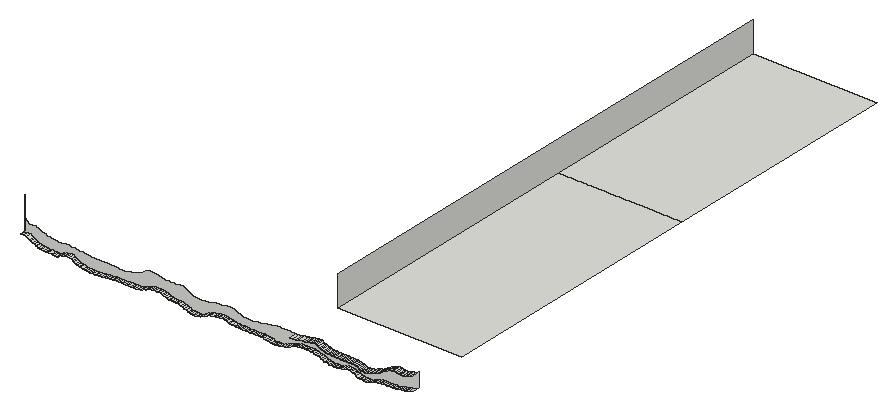
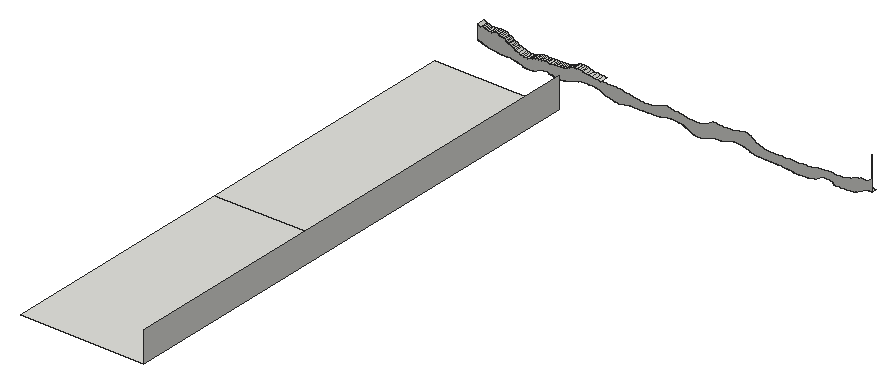
# SketchUp Ruby script. Lengths in inches.
U = 1.inch
M = Sketchup.active_model
def pt(a) = Geom::Point3d.new(a.map { |v| v * U })
def face(e, loops, mat)
  f = e.add_face(loops[0].map { |a| pt(a) })
  loops[1..].each { |l| e.add_face(l.map { |a| pt(a) }).erase! }
  f.material = f.back_material = mat if mat
  f
end
# faces: each face lists its corners as indices into pts; further lists are holes
def faces(e, pts, list, mat = nil) = list.each { |f| face(e, (f[0].is_a?(Array) ? f : [f]).map { |l| l.map { |i| pts[i] } }, mat) }
# xy, xz, yz: faces in a plane at the given z, y or x. An outline is a flat list of corners, or four numbers for a rectangle; further outlines are holes
def ring(l) = l.size == 4 ? [[l[0], l[1]], [l[2], l[1]], [l[2], l[3]], [l[0], l[3]]] : l.each_slice(2).to_a
def flat(e, list, mat, &to3) = list.each { |f| face(e, (f[0].is_a?(Array) ? f : [f]).map { |l| ring(l).map { |u, v| to3.(u, v) } }, mat) }
def xy(e, z, list, mat = nil) = flat(e, list, mat) { |x, y| [x, y, z] }
def xz(e, y, list, mat = nil) = flat(e, list, mat) { |x, z| [x, y, z] }
def yz(e, x, list, mat = nil) = flat(e, list, mat) { |y, z| [x, y, z] }
def lines(e, pts, list) = list.each { |a, b| e.add_line(pt(pts[a]), pt(pts[b])) }
# prism: a flat outline (further loops are holes) pulled along v
def prism(e, loops, v, mat = nil)
  f = face(e, loops, mat); d = Geom::Vector3d.new(v.map { |x| x * U })
  f.pushpull(f.normal.samedirection?(d) ? d.length : -d.length)
end
def box(e, o, s, mat = nil) = prism(e, [[o, [o[0] + s[0], o[1], o[2]], [o[0] + s[0], o[1] + s[1], o[2]], [o[0], o[1] + s[1], o[2]]]], [0, 0, s[2]], mat)
def at(x, y, z, deg = 0) = Geom::Transformation.translation(pt([x, y, z])) * Geom::Transformation.rotation(ORIGIN, Z_AXIS, deg.degrees)
def axes(o, x, y, z) = Geom::Transformation.new([*x, 0, *y, 0, *z, 0, *pt(o).to_a, 1])
def part(name) = M.definitions.add(name)
# library, detail: a bought-in or finely detailed component or shape, given as its bounding box
def library(name, o, s) = part(name).tap { |d| box(d.entities, o, s) }
def detail(e, o, s) = box(e.add_group.entities, o, s)
def put(e, d, t, mat = nil) = e.add_instance(d, t).tap { |i| i.material = mat if mat }
def group(e, t, mat = nil) = e.add_group.tap { |g| g.transformation = t; g.material = mat if mat }.entities
root = M.entities
xy(root,237.65,[[282.08,566.68,282.77,568.68],[282.77,566.68,283.39,568.68]])
xy(root,238.18,[[376.03,566.68,376.71,568.68]])
xy(root,238.33,[[291.18,566.68,291.73,568.68],[291.73,566.68,292.41,568.68]])
xy(root,238.34,[[293.09,566.68,294.02,568.68],[294.02,566.68,294.51,568.68],[294.51,566.68,295.27,568.68],[295.27,566.68,295.9,568.68],[295.9,566.68,296.65,568.68],
  [296.65,566.68,297.27,568.68],[297.27,566.68,298.04,568.68],[298.04,566.68,298.66,568.68]])
xy(root,238.62,[[342.56,566.68,343.33,568.68],[343.33,566.68,343.96,568.68],[343.96,566.68,344.72,568.68],[344.72,566.68,345.34,568.68],[345.34,566.68,346.19,568.68],
  [346.19,566.68,346.83,568.68],[346.83,566.68,347.45,568.68]])
xy(root,238.625,[[341.14,566.68,342,568.68]])
xy(root,238.89,[[396.95,566.68,397.63,568.68]])
xy(root,238.9,[[398.39,566.68,399.01,568.68],[399.01,566.68,399.78,568.68]])
xy(root,240.43,[[365.23,566.68,365.8,568.68]])
xy(root,241.52,[[252.78,566.68,252.84,568.68]])
xy(root,242.28,[[383.05,565.74,383.5625,568.68]])
xy(root,242.3,[[381.29,565.74,381.96,568.68]])
xy(root,242.33,[[378.88,565.74,379.46,568.68]])
xy(root,242.625,[[358.39,589.83,406.85,697.21],[358.39,697.21,406.85,792.52]])
xz(root,568.68,[[321.7,236.98,321.09,237.01,320.4,237.04,319.64,237.11,318.95,237.2,318.42,237.33,317.75,237.68,316.8125,237.96,316.25,238.28,315.47,238.43,314.69,238.78,314.02,238.79,313.48,238.8,312.72,238.83,311.97,238.875,311.4,238.94,310.82,239.04,310.16,239.29,309.58,239.53,309.05,239.7,308.36,239.92,307.73,240.11,306.95,240.27,306.33,240.25,305.625,240.23,304.86,240.19,304.1875,240.12,303.53,240.03,302.89,239.85,302.34,239.52,301.78,239.35,301.19,239.18,300.68,238.86,299.99,238.72,299.17,238.59,298.66,238.34,293.09,238.34,292.41,238.33,291.18,238.33,290.46,238.32,289.61,238.3,288.98,238.28,288.23,238.26,287.6,238.15,286.84,238.13,286.29,238.1,285.4375,237.98,284.82,237.94,284.06,237.89,283.39,237.65,282.08,237.65,281.39,237.66,280.64,237.67,280.04,237.68,279.43,237.71,278.72,237.76,278.03,237.82,277.37,237.9,276.43,238.21,275.96,238.31,275.05,238.43,274.4,238.74,273.82,239.11,273.24,239.38,272.78,239.71,272.08,240.11,271.39,240.09,270.73,240.05,270.14,239.99,269.41,239.88,268.86,239.69,268.28,239.55,267.72,238.9375,267.19,238.77,266.45,238.79,265.58,238.8,265.07,238.82,264.03,238.92,263.34,238.93,262.64,238.94,261.94,238.97,261.26,239.03,260.57,239.09,259.79,239.19,259.28,239.52,258.72,239.64,258.27,239.86,257.48,240.2,256.88,240.59,256.34,240.85,255.32,241.55,254.05,241.69,252.84,241.52,252.84,246.2,254.41,244.96,255.8,244.9375,257.05,244.92,257.27,244.61,257.83,244.54,258.59,244.41,259.26,244.11,259.78,243.95,260.44,243.79,260.96,243.48,261.6,243.3,262.1875,243.14,262.67,243.06,263.39,242.85,263.97,242.78,264.78,242.73,265.32,242.68,265.99,242.51,266.51,242.46,267.05,242.58,267.68,242.57,268.31,242.81,268.88,242.86,269.44,242.89,270.08,242.92,270.51,242.625,271.12,242.65,271.67,242.62,272.3,242.58,272.86,242.57,273.5,242.48,274.16,242.38,274.82,242.34,275.49,242.24,276.66,241.96,277.43,241.89,278.25,241.83,278.85,241.78,279.62,241.75,280.07,241.74,280.62,241.72,281.88,241.7,282.61,241.69,283.28,241.68,283.87,241.68,284.36,241.67,285.0625,241.74,285.63,241.75,287.63,241.75,288.12,241.67,288.65,241.66,289.26,241.57,289.8,241.53,290.42,241.51,290.97,241.49,291.67,241.48,292.33,241.47,292.9,241.46,293.61,241.6,294.34,241.85,295.01,241.91,295.91,242.1,296.68,242.46,297.38,242.78,298.15,242.97,298.68,243.23,299.08,243.48,299.6,243.72,299.9375,244.12,300.41,244.39,300.89,244.73,301.375,244.87,301.96,244.95,302.64,245.01,303.29,244.81,303.86,244.7,304.34,244.67,304.95,244.55,305.49,244.51,305.95,244.25,306.7,244.11,307.26,244.04,307.88,243.99,308.6,243.95,309.1,243.93,309.79,243.91,310.36,243.89,311.06,243.88,311.71,243.94,312.35,243.95,312.91,244.1,313.54,244.13,314.02,244.15,314.54,244.17,315.06,244.18,315.66,243.8,316.2,243.43,316.81,243.09,317.2,242.875,317.7,242.68,318.29,242.51,318.8,242.21,319.4,242.11,320.08,241.96,320.64,241.89,321.1,241.85,321.62,241.8125,322.13,241.79,322.71,241.78,323.38,241.91,323.85,241.93,324.52,242.09,325.29,242.2,325.79,242.24,326.4,242.42,326.95,242.47,327.7,242.71,328.34,242.78,328.82,242.82,329.51,242.85,330.21,242.87,330.76,243.02,331.38,243.05,331.93,243.29,332.61,243.35,333.16,243.39,333.76,243.42,334.53,243.14,335.1,242.9375,335.65,242.65,336.27,242.39,337.03,242.14,337.67,241.89,338.16,241.78,339.21,241.63,339.98,241.56,340.58,241.51,341.03,241.48,341.55,241.46,342.42,241.51,343.14,241.59,344.08,241.82,344.86,241.87,345.625,241.98,346.24,242.02,346.89,242.19,347.59,242.38,348.08,242.4375,348.6,242.48,349.26,242.58,349.79,242.61,350.375,242.77,350.83,242.95,351.39,243.01,351.9,243.05,352.47,243.08,353.125,243.09,355.28,243.09,355.85,243.08,356.4375,243.07,357.02,243.07,357.68,243.0625,358.29,243.05,358.97,243.05,360.24,243.1,361.41,243.17,362.55,243.4,363.8125,243.52,364.94,243.71,365.84,243.99,366.54,244.08,367.24,244.21,367.82,244.27,368.36,244.3,369.03,244.39,369.625,244.19,370,243.88,370.48,243.59,371.03,243.33,371.58,243.22,372.07,242.92,372.55,242.75,373.11,242.6,373.67,242.52,374.23,242.47,374.8125,242.43,375.39,242.4,375.97,242.39,376.55,242.37,377.13,242.36,377.72,242.35,378.88,242.33,379.46,242.33,380.18,242.32,380.65,242.3125,381.29,242.3,381.96,242.3,382.41,242.29,383.05,242.28,383.5625,242.28,384.19,242.2,384.77,241.97,385.34,241.84,385.85,241.57,386.27,241.33,386.74,241.24,387.27,241.17,387.74,241.12,388.34,241.09,388.91,241.14,389.55,241.35,390.14,241.46,391.08,241.85,392.08,242.23,392.64,242.42,393.36,242.61,393.875,242.91,394.25,243.14,394.79,243.52,395.27,243.71,395.6,244.02,396.04,244.21,396.63,244.57,397.1,244.76,397.72,245.125,398.22,245.32,398.7,245.41,399.25,245.48,399.74,245.59,400.27,245.55,400.88,245.35,401.37,245.31,401.92,245.27,402.48,245.24,403.04,245.22,403.6,245.34,404.23,245.42,404.8125,245.52,405.19,245.76,405.66,245.9,406.85,246.43,406.85,240.89,405.02,240.1,404.46,239.96,403.9375,239.81,403.25,239.53,402.7,239.49,401.98,239.42,401.18,239.28,400.41,239.15,399.78,238.9,398.39,238.9,397.63,238.89,396.95,238.89,396.27,238.88,395.73,238.875,394.97,238.86,394.23,238.83,393.66,238.8,393.08,238.74,392.42,238.6,391.85,238.51,391.32,238.33,390.63,238.08,389.95,237.84,389.26,237.5625,388.66,237.47,387.98,237.4,387.25,237.42,386.68,237.45,386.09,237.51,385.49,237.59,384.95,237.71,384.12,238,383.41,238.33,382.86,238.57,382.36,238.86,381.84,238.96,381.15,239.02,380.47,239.125,379.73,239.04,379.16,238.66,378.57,238.61,377.91,238.55,377.39,238.27,376.71,238.18,376.03,238.18,375.36,238.11,374.83,238.15,374.01,238.19,373.4375,238.26,372.87,238.48,372.21,238.56,371.64,238.67,371.12,239.01,370.4375,239.18,369.8125,239.5,369.05,239.65,368.4375,239.8,367.68,239.96,367.03,240.23,366.45,240.27,365.8,240.43,365.23,240.43,364.65,240.42,364.125,240.41,363.43,240.4,362.74,240.37,362.05,240.33,361.37,240.27,360.69,240.17,360.07,239.97,359.42,239.75,358.68,239.375,357.89,239.08,357.01,238.72,356.26,238.46,355.04,238.14,353.92,237.88,353.27,237.87,352.4,237.74,351.69,237.79,350.92,237.86,350.29,238.15,349.52,238.19,348.9,238.25,348.14,238.45,347.45,238.62,342.56,238.62,342,238.625,341.14,238.625,340.45,238.63,339.83,238.64,339.05,238.65,338.38,238.66,337.69,238.6875,337.02,238.73,336.54,238.78,335.66,238.93,334.89,239.07,334.34,239.16,333.49,239.44,332.82,239.56,332.21,239.72,331.48,239.7,330.92,239.69,330.33,239.65,329.71,239.6,329.22,239.54,328.41,239.31,327.41,239.22,326.83,239.12,326.1875,238.76,325.55,238.51,324.99,238.375,324.55,238.02,323.85,237.74,323.23,237.43,322.38,237.22],[252.78,241.52,252.84,254.5]])
yz(root,358.39,[[589.83,242.625,792.52,254.5]])
p = [[319.64,568.68,237.11],[320.4,568.68,237.04],[320.4,566.68,237.04],[319.64,566.68,237.11],[321.09,568.68,237.01],[321.09,566.68,237.01],
  [321.7,568.68,236.98],[321.7,566.68,236.98],[322.38,568.68,237.22],[322.38,566.68,237.22],[318.95,568.68,237.2],[318.95,566.68,237.2],
  [318.42,568.68,237.33],[318.42,566.68,237.33],[323.23,568.68,237.43],[323.23,566.68,237.43],[317.75,568.68,237.68],[317.75,566.68,237.68],
  [323.85,568.68,237.74],[323.85,566.68,237.74],[386.68,568.68,237.45],[387.25,568.68,237.42],[387.25,566.68,237.42],[386.68,566.68,237.45],
  [387.98,568.68,237.4],[387.98,566.68,237.4],[388.66,568.68,237.47],[388.66,566.68,237.47],[385.49,568.68,237.59],[386.09,568.68,237.51],
  [386.09,566.68,237.51],[385.49,566.68,237.59],[389.26,568.68,237.5625],[389.26,566.68,237.5625],[283.39,568.68,237.65],[284.06,568.68,237.89],
  [284.06,566.68,237.89],[283.39,566.68,237.65],[384.95,568.68,237.71],[384.95,566.68,237.71],[389.95,568.68,237.84],[389.95,566.68,237.84],
  [278.72,568.68,237.76],[279.43,568.68,237.71],[279.43,566.68,237.71],[278.72,566.68,237.76],[280.04,568.68,237.68],[280.04,566.68,237.68],
  [280.64,568.68,237.67],[280.64,566.68,237.67],[281.39,568.68,237.66],[281.39,566.68,237.66],[282.08,568.68,237.65],[282.08,566.68,237.65],
  [316.8125,568.68,237.96],[316.8125,566.68,237.96],[324.55,568.68,238.02],[324.55,566.68,238.02],[351.69,568.68,237.79],[352.4,568.68,237.74],
  [352.4,566.68,237.74],[351.69,566.68,237.79],[353.27,568.68,237.87],[353.27,566.68,237.87],[384.12,568.68,238],[384.12,566.68,238],
  [277.37,568.68,237.9],[278.03,568.68,237.82],[278.03,566.68,237.82],[277.37,566.68,237.9],[350.92,568.68,237.86],[350.92,566.68,237.86],
  [390.63,568.68,238.08],[390.63,566.68,238.08],[276.43,568.68,238.21],[276.43,566.68,238.21],[284.82,568.68,237.94],[284.82,566.68,237.94],
  [285.4375,568.68,237.98],[285.4375,566.68,237.98],[350.29,568.68,238.15],[350.29,566.68,238.15],[353.92,568.68,237.88],[353.92,566.68,237.88],
  [355.04,568.68,238.14],[355.04,566.68,238.14],[286.29,568.68,238.1],[286.29,566.68,238.1],[316.25,568.68,238.28],[316.25,566.68,238.28],
  [324.99,568.68,238.375],[324.99,566.68,238.375],[383.41,568.68,238.33],[383.41,566.68,238.33],[286.84,568.68,238.13],[286.84,566.68,238.13],
  [287.6,568.68,238.15],[287.6,566.68,238.15],[349.52,568.68,238.19],[349.52,566.68,238.19],[356.26,568.68,238.46],[356.26,566.68,238.46],
  [374.01,568.68,238.19],[374.83,568.68,238.15],[374.83,566.68,238.15],[374.01,566.68,238.19],[375.36,568.68,238.11],[375.36,566.68,238.11],
  [376.03,568.68,238.18],[376.03,566.68,238.18],[391.32,568.68,238.33],[391.32,566.68,238.33],[275.96,568.68,238.31],[275.96,566.68,238.31],
  [288.23,568.68,238.26],[288.23,566.68,238.26],[348.9,568.68,238.25],[348.9,566.68,238.25],[373.4375,568.68,238.26],[373.4375,566.68,238.26],
  [376.71,568.68,238.18],[377.39,568.68,238.27],[377.39,566.68,238.27],[376.71,566.68,238.18],[275.05,568.68,238.43],[275.05,566.68,238.43],
  [288.98,568.68,238.28],[288.98,566.68,238.28],[289.61,568.68,238.3],[289.61,566.68,238.3],[290.46,568.68,238.32],[290.46,566.68,238.32],
  [291.18,568.68,238.33],[291.18,566.68,238.33],[292.41,568.68,238.33],[293.09,568.68,238.34],[293.09,566.68,238.34],[292.41,566.68,238.33],
  [298.66,568.68,238.34],[299.17,568.68,238.59],[299.17,566.68,238.59],[298.66,566.68,238.34],[315.47,568.68,238.43],[315.47,566.68,238.43],
  [348.14,568.68,238.45],[348.14,566.68,238.45],[372.87,568.68,238.48],[372.87,566.68,238.48],[377.91,568.68,238.55],[377.91,566.68,238.55],
  [382.86,568.68,238.57],[382.86,566.68,238.57],[391.85,568.68,238.51],[391.85,566.68,238.51],[274.4,568.68,238.74],[274.4,566.68,238.74],
  [314.69,568.68,238.78],[314.69,566.68,238.78],[325.55,568.68,238.51],[325.55,566.68,238.51],[326.1875,568.68,238.76],[326.1875,566.68,238.76],
  [347.45,568.68,238.62],[347.45,566.68,238.62],[357.01,568.68,238.72],[357.01,566.68,238.72],[372.21,568.68,238.56],[372.21,566.68,238.56],
  [378.57,568.68,238.61],[378.57,566.68,238.61],[392.42,568.68,238.6],[392.42,566.68,238.6],[299.99,568.68,238.72],[299.99,566.68,238.72],
  [338.38,568.68,238.66],[339.05,568.68,238.65],[339.05,566.68,238.65],[338.38,566.68,238.66],[339.83,568.68,238.64],[339.83,566.68,238.64],
  [340.45,568.68,238.63],[340.45,566.68,238.63],[341.14,568.68,238.625],[341.14,566.68,238.625],[342,568.68,238.625],[342.56,568.68,238.62],
  [342.56,566.68,238.62],[342,566.68,238.625],[371.64,568.68,238.67],[371.64,566.68,238.67],[379.16,568.68,238.66],[379.16,566.68,238.66],
  [382.36,568.68,238.86],[382.36,566.68,238.86],[393.08,568.68,238.74],[393.08,566.68,238.74],[273.82,568.68,239.11],[273.82,566.68,239.11],
  [300.68,568.68,238.86],[300.68,566.68,238.86],[336.54,568.68,238.78],[337.02,568.68,238.73],[337.02,566.68,238.73],[336.54,566.68,238.78],
  [337.69,568.68,238.6875],[337.69,566.68,238.6875],[357.89,568.68,239.08],[357.89,566.68,239.08],[371.12,568.68,239.01],[371.12,566.68,239.01],
  [379.73,568.68,239.04],[379.73,566.68,239.04],[393.66,568.68,238.8],[393.66,566.68,238.8],[264.03,568.68,238.92],[265.07,568.68,238.82],
  [265.07,566.68,238.82],[264.03,566.68,238.92],[265.58,568.68,238.8],[265.58,566.68,238.8],[266.45,568.68,238.79],[266.45,566.68,238.79],
  [267.19,568.68,238.77],[267.19,566.68,238.77],[267.72,568.68,238.9375],[267.72,566.68,238.9375],[311.97,568.68,238.875],[312.72,568.68,238.83],
  [312.72,566.68,238.83],[311.97,566.68,238.875],[313.48,568.68,238.8],[313.48,566.68,238.8],[314.02,568.68,238.79],[314.02,566.68,238.79],
  [326.83,568.68,239.12],[326.83,566.68,239.12],[335.66,568.68,238.93],[335.66,566.68,238.93],[394.23,568.68,238.83],[394.23,566.68,238.83],
  [394.97,568.68,238.86],[394.97,566.68,238.86],[261.94,568.68,238.97],[262.64,568.68,238.94],[262.64,566.68,238.94],[261.94,566.68,238.97],
  [263.34,568.68,238.93],[263.34,566.68,238.93],[268.28,568.68,239.55],[268.28,566.68,239.55],[301.19,568.68,239.18],[301.19,566.68,239.18],
  [310.82,568.68,239.04],[311.4,568.68,238.94],[311.4,566.68,238.94],[310.82,566.68,239.04],[334.89,568.68,239.07],[334.89,566.68,239.07],
  [381.84,568.68,238.96],[381.84,566.68,238.96],[395.73,568.68,238.875],[395.73,566.68,238.875],[396.27,568.68,238.88],[396.27,566.68,238.88],
  [396.95,568.68,238.89],[396.95,566.68,238.89],[397.63,568.68,238.89],[398.39,568.68,238.9],[398.39,566.68,238.9],[397.63,566.68,238.89],
  [399.78,568.68,238.9],[400.41,568.68,239.15],[400.41,566.68,239.15],[399.78,566.68,238.9],[260.57,568.68,239.09],[261.26,568.68,239.03],
  [261.26,566.68,239.03],[260.57,566.68,239.09],[310.16,568.68,239.29],[310.16,566.68,239.29],[370.4375,568.68,239.18],[370.4375,566.68,239.18],
  [380.47,568.68,239.125],[380.47,566.68,239.125],[381.15,568.68,239.02],[381.15,566.68,239.02],[259.79,568.68,239.19],[259.79,566.68,239.19],
  [273.24,568.68,239.38],[273.24,566.68,239.38],[327.41,568.68,239.22],[327.41,566.68,239.22],[334.34,568.68,239.16],[334.34,566.68,239.16],
  [358.68,568.68,239.375],[358.68,566.68,239.375],[259.28,568.68,239.52],[259.28,566.68,239.52],[301.78,568.68,239.35],[301.78,566.68,239.35],
  [328.41,568.68,239.31],[328.41,566.68,239.31],[333.49,568.68,239.44],[333.49,566.68,239.44],[369.8125,568.68,239.5],[369.8125,566.68,239.5],
  [401.18,568.68,239.28],[401.18,566.68,239.28],[309.58,568.68,239.53],[309.58,566.68,239.53],[329.22,568.68,239.54],[329.22,566.68,239.54],
  [401.98,568.68,239.42],[401.98,566.68,239.42],[272.78,568.68,239.71],[272.78,566.68,239.71],[302.34,568.68,239.52],[302.34,566.68,239.52],
  [332.82,568.68,239.56],[332.82,566.68,239.56],[359.42,568.68,239.75],[359.42,566.68,239.75],[402.7,568.68,239.49],[402.7,566.68,239.49],
  [258.72,568.68,239.64],[258.72,566.68,239.64],[302.89,568.68,239.85],[302.89,566.68,239.85],[309.05,568.68,239.7],[309.05,566.68,239.7],
  [329.71,568.68,239.6],[329.71,566.68,239.6],[369.05,568.68,239.65],[369.05,566.68,239.65],[403.25,568.68,239.53],[403.25,566.68,239.53],
  [403.9375,568.68,239.81],[403.9375,566.68,239.81],[258.27,568.68,239.86],[258.27,566.68,239.86],[268.86,568.68,239.69],[268.86,566.68,239.69],
  [330.33,568.68,239.65],[330.33,566.68,239.65],[330.92,568.68,239.69],[330.92,566.68,239.69],[332.21,568.68,239.72],[332.21,566.68,239.72],
  [269.41,568.68,239.88],[269.41,566.68,239.88],[272.08,568.68,240.11],[272.08,566.68,240.11],[308.36,568.68,239.92],[308.36,566.68,239.92],
  [331.48,568.68,239.7],[331.48,566.68,239.7],[360.07,568.68,239.97],[360.07,566.68,239.97],[368.4375,568.68,239.8],[368.4375,566.68,239.8],
  [303.53,568.68,240.03],[303.53,566.68,240.03],[367.68,568.68,239.96],[367.68,566.68,239.96],[404.46,568.68,239.96],[404.46,566.68,239.96],
  [257.48,568.68,240.2],[257.48,566.68,240.2],[270.14,568.68,239.99],[270.14,566.68,239.99],[307.73,568.68,240.11],[307.73,566.68,240.11],
  [270.73,568.68,240.05],[270.73,566.68,240.05],[271.39,568.68,240.09],[271.39,566.68,240.09],[304.1875,568.68,240.12],[304.1875,566.68,240.12],
  [360.69,568.68,240.17],[360.69,566.68,240.17],[367.03,568.68,240.23],[367.03,566.68,240.23],[405.02,568.68,240.1],[405.02,566.68,240.1],
  [304.86,568.68,240.19],[304.86,566.68,240.19],[306.95,568.68,240.27],[306.95,566.68,240.27],[406.85,568.68,240.89],[406.85,566.68,240.89],
  [256.88,568.68,240.59],[256.88,566.68,240.59],[305.625,568.68,240.23],[305.625,566.68,240.23],[306.33,568.68,240.25],[306.33,566.68,240.25],
  [361.37,568.68,240.27],[361.37,566.68,240.27],[366.45,568.68,240.27],[366.45,566.68,240.27],[362.05,568.68,240.33],[362.05,566.68,240.33],
  [362.74,568.68,240.37],[362.74,566.68,240.37],[365.8,568.68,240.43],[365.8,566.68,240.43],[363.43,568.68,240.4],[363.43,566.68,240.4],
  [364.125,568.68,240.41],[364.125,566.68,240.41],[364.65,568.68,240.42],[364.65,566.68,240.42],[365.23,568.68,240.43],[365.23,566.68,240.43],
  [256.34,568.68,240.85],[256.34,566.68,240.85],[255.32,568.68,241.55],[255.32,566.68,241.55],[387.27,568.68,241.17],[387.74,568.68,241.12],
  [387.74,565.74,241.12],[387.27,565.74,241.17],[388.34,568.68,241.09],[388.34,565.74,241.09],[388.91,568.68,241.14],[388.91,565.74,241.14],
  [389.55,568.68,241.35],[389.55,565.74,241.35],[386.27,568.68,241.33],[386.74,568.68,241.24],[386.74,565.74,241.24],[386.27,565.74,241.33],
  [385.85,568.68,241.57],[385.85,565.74,241.57],[390.14,568.68,241.46],[390.14,565.74,241.46],[391.08,568.68,241.85],[391.08,565.74,241.85],
  [252.84,568.68,241.52],[254.05,568.68,241.69],[254.05,566.68,241.69],[252.84,566.68,241.52],[385.34,568.68,241.84],[385.34,565.74,241.84],
  [384.77,568.68,241.97],[384.77,565.74,241.97],[392.08,568.68,242.23],[392.08,565.74,242.23],[384.19,568.68,242.2],[384.19,565.74,242.2],
  [383.5625,568.68,242.28],[383.5625,565.74,242.28],[392.64,568.68,242.42],[392.64,565.74,242.42],[377.72,568.68,242.35],[378.3,568.68,242.34],
  [378.3,565.74,242.34],[377.72,565.74,242.35],[378.88,568.68,242.33],[378.88,565.74,242.33],[379.46,568.68,242.33],[380.18,568.68,242.32],
  [380.18,565.74,242.32],[379.46,565.74,242.33],[380.65,568.68,242.3125],[380.65,565.74,242.3125],[381.29,568.68,242.3],[381.29,565.74,242.3],
  [381.96,568.68,242.3],[382.41,568.68,242.29],[382.41,565.74,242.29],[381.96,565.74,242.3],[383.05,568.68,242.28],[383.05,565.74,242.28],
  [374.23,568.68,242.47],[374.8125,568.68,242.43],[374.8125,565.74,242.43],[374.23,565.74,242.47],[375.39,568.68,242.4],[375.39,565.74,242.4],
  [375.97,568.68,242.39],[375.97,565.74,242.39],[376.55,568.68,242.37],[376.55,565.74,242.37],[377.13,568.68,242.36],[377.13,565.74,242.36],
  [393.36,568.68,242.61],[393.36,565.74,242.61],[373.11,568.68,242.6],[373.67,568.68,242.52],[373.67,565.74,242.52],[373.11,565.74,242.6],
  [372.55,568.68,242.75],[372.55,565.74,242.75],[393.875,568.68,242.91],[393.875,565.74,242.91],[372.07,568.68,242.92],[372.07,565.74,242.92],
  [371.58,568.68,243.22],[371.58,565.74,243.22],[394.25,568.68,243.14],[394.25,565.74,243.14],[358.97,568.68,243.05],[360.24,568.68,243.1],
  [360.24,565.74,243.1],[358.97,565.74,243.05],[361.41,568.68,243.17],[361.41,565.74,243.17],[394.79,568.68,243.52],[394.79,565.74,243.52],
  [362.55,568.68,243.4],[362.55,565.74,243.4],[371.03,568.68,243.33],[371.03,565.74,243.33],[370.48,568.68,243.59],[370.48,565.74,243.59],
  [363.8125,568.68,243.52],[363.8125,565.74,243.52],[364.94,568.68,243.71],[364.94,565.74,243.71],[395.27,568.68,243.71],[395.27,565.74,243.71],
  [370,568.68,243.88],[370,565.74,243.88],[365.84,568.68,243.99],[365.84,565.74,243.99],[395.6,568.68,244.02],[395.6,565.74,244.02],
  [369.625,568.68,244.19],[369.625,565.74,244.19],[366.54,568.68,244.08],[366.54,565.74,244.08],[396.04,568.68,244.21],[396.04,565.74,244.21],
  [367.24,568.68,244.21],[367.24,565.74,244.21],[367.82,568.68,244.27],[367.82,565.74,244.27],[369.03,568.68,244.39],[369.03,565.74,244.39],
  [396.63,568.68,244.57],[396.63,565.74,244.57],[368.36,568.68,244.3],[368.36,565.74,244.3],[397.1,568.68,244.76],[397.1,565.74,244.76],
  [397.72,568.68,245.125],[397.72,565.74,245.125],[398.22,568.68,245.32],[398.22,565.74,245.32],[401.92,568.68,245.27],[402.48,568.68,245.24],
  [402.48,565.74,245.24],[401.92,565.74,245.27],[403.04,568.68,245.22],[403.04,565.74,245.22],[403.6,568.68,245.34],[403.6,565.74,245.34],
  [398.7,568.68,245.41],[398.7,565.74,245.41],[400.27,568.68,245.55],[400.88,568.68,245.35],[400.88,565.74,245.35],[400.27,565.74,245.55],
  [401.37,568.68,245.31],[401.37,565.74,245.31],[404.23,568.68,245.42],[404.23,565.74,245.42],[399.25,568.68,245.48],[399.25,565.74,245.48],
  [404.8125,568.68,245.52],[404.8125,565.74,245.52],[399.74,568.68,245.59],[399.74,565.74,245.59],[405.19,568.68,245.76],[405.19,565.74,245.76],
  [405.66,568.68,245.9],[405.66,565.74,245.9],[406.85,568.68,246.43],[406.85,565.74,246.43]]
faces(root,p,[[0,1,2,3],[1,4,5,2],[4,6,7,5],[6,8,9,7],[10,0,3,11],[12,10,11,13],[8,14,15,9],[16,12,13,17],
  [14,18,19,15],[20,21,22,23],[21,24,25,22],[24,26,27,25],[28,29,30,31],[29,20,23,30],[26,32,33,27],[34,35,36,37],
  [38,28,31,39],[32,40,41,33],[42,43,44,45],[43,46,47,44],[46,48,49,47],[48,50,51,49],[50,52,53,51],[54,16,17,55],
  [18,56,57,19],[58,59,60,61],[59,62,63,60],[64,38,39,65],[66,67,68,69],[67,42,45,68],[70,58,61,71],[40,72,73,41],
  [74,66,69,75],[35,76,77,36],[76,78,79,77],[80,70,71,81],[62,82,83,63],[82,84,85,83],[78,86,87,79],[88,54,55,89],
  [56,90,91,57],[92,64,65,93],[86,94,95,87],[94,96,97,95],[98,80,81,99],[84,100,101,85],[102,103,104,105],[103,106,107,104],
  [106,108,109,107],[72,110,111,73],[112,74,75,113],[96,114,115,97],[116,98,99,117],[118,102,105,119],[120,121,122,123],[124,112,113,125],
  [114,126,127,115],[126,128,129,127],[128,130,131,129],[130,132,133,131],[134,135,136,137],[138,139,140,141],[142,88,89,143],[144,116,117,145],
  [146,118,119,147],[121,148,149,122],[150,92,93,151],[110,152,153,111],[154,124,125,155],[156,142,143,157],[90,158,159,91],[158,160,161,159],
  [162,144,145,163],[100,164,165,101],[166,146,147,167],[148,168,169,149],[152,170,171,153],[139,172,173,140],[174,175,176,177],[175,178,179,176],
  [178,180,181,179],[180,182,183,181],[184,185,186,187],[188,166,167,189],[168,190,191,169],[192,150,151,193],[170,194,195,171],[196,154,155,197],
  [172,198,199,173],[200,201,202,203],[201,204,205,202],[204,174,177,205],[164,206,207,165],[208,188,189,209],[190,210,211,191],[194,212,213,195],
  [214,215,216,217],[215,218,219,216],[218,220,221,219],[220,222,223,221],[222,224,225,223],[226,227,228,229],[227,230,231,228],[230,232,233,231],
  [232,156,157,233],[160,234,235,161],[236,200,203,237],[212,238,239,213],[238,240,241,239],[242,243,244,245],[243,246,247,244],[246,214,217,247],
  [224,248,249,225],[198,250,251,199],[252,253,254,255],[253,226,229,254],[256,236,237,257],[258,192,193,259],[240,260,261,241],[260,262,263,261],
  [262,264,265,263],[266,267,268,269],[270,271,272,273],[274,275,276,277],[275,242,245,276],[278,252,255,279],[280,208,209,281],[210,282,283,211],
  [282,284,285,283],[284,258,259,285],[286,274,277,287],[288,196,197,289],[234,290,291,235],[292,256,257,293],[206,294,295,207],[296,286,287,297],
  [250,298,299,251],[290,300,301,291],[302,292,293,303],[304,280,281,305],[271,306,307,272],[308,278,279,309],[300,310,311,301],[306,312,313,307],
  [314,288,289,315],[298,316,317,299],[318,302,303,319],[294,320,321,295],[312,322,323,313],[324,296,297,325],[316,326,327,317],[328,308,309,329],
  [310,330,331,311],[332,304,305,333],[322,334,335,323],[334,336,337,335],[338,324,325,339],[248,340,341,249],[330,342,343,331],[342,344,345,343],
  [346,318,319,347],[340,348,349,341],[350,314,315,351],[352,328,329,353],[344,354,355,345],[354,346,347,355],[320,356,357,321],[358,332,333,359],
  [326,360,361,327],[362,358,359,363],[336,364,365,337],[366,338,339,367],[348,368,369,349],[370,352,353,371],[368,372,373,369],[372,374,375,373],
  [360,376,377,361],[356,378,379,357],[380,362,363,381],[364,382,383,365],[374,350,351,375],[376,384,385,377],[386,370,371,387],[382,388,389,383],
  [390,366,367,391],[384,392,393,385],[392,394,395,393],[378,396,397,379],[398,380,381,399],[394,386,387,395],[396,400,401,397],[400,402,403,401],
  [404,398,399,405],[402,406,407,403],[406,408,409,407],[408,410,411,409],[410,412,413,411],[414,390,391,415],[416,414,415,417],[418,419,420,421],
  [419,422,423,420],[422,424,425,423],[424,426,427,425],[428,429,430,431],[429,418,421,430],[432,428,431,433],[426,434,435,427],[434,436,437,435],
  [438,439,440,441],[442,432,433,443],[439,416,417,440],[444,442,443,445],[436,446,447,437],[448,444,445,449],[450,448,449,451],[446,452,453,447],
  [454,455,456,457],[455,458,459,456],[460,461,462,463],[461,464,465,462],[464,466,467,465],[468,469,470,471],[469,472,473,470],[474,475,476,477],
  [475,478,479,476],[478,480,481,479],[480,482,483,481],[482,484,485,483],[484,454,457,485],[452,486,487,453],[488,489,490,491],[489,474,477,490],
  [492,488,491,493],[486,494,495,487],[496,492,493,497],[498,496,497,499],[494,500,501,495],[502,503,504,505],[503,506,507,504],[500,508,509,501],
  [506,510,511,507],[512,498,499,513],[514,512,513,515],[510,516,517,511],[516,518,519,517],[508,520,521,509],[522,514,515,523],[518,524,525,519],
  [520,526,527,521],[528,522,523,529],[524,530,531,525],[526,532,533,527],[530,534,535,531],[534,536,537,535],[538,528,529,539],[532,540,541,533],
  [536,542,543,537],[542,538,539,543],[540,544,545,541],[544,546,547,545],[546,548,549,547],[550,551,552,553],[551,554,555,552],[554,556,557,555],
  [548,558,559,549],[560,561,562,563],[561,564,565,562],[564,550,553,565],[556,566,567,557],[558,568,569,559],[566,570,571,567],[568,572,573,569],
  [570,574,575,571],[572,560,563,573],[574,576,577,575],[576,578,579,577]])
